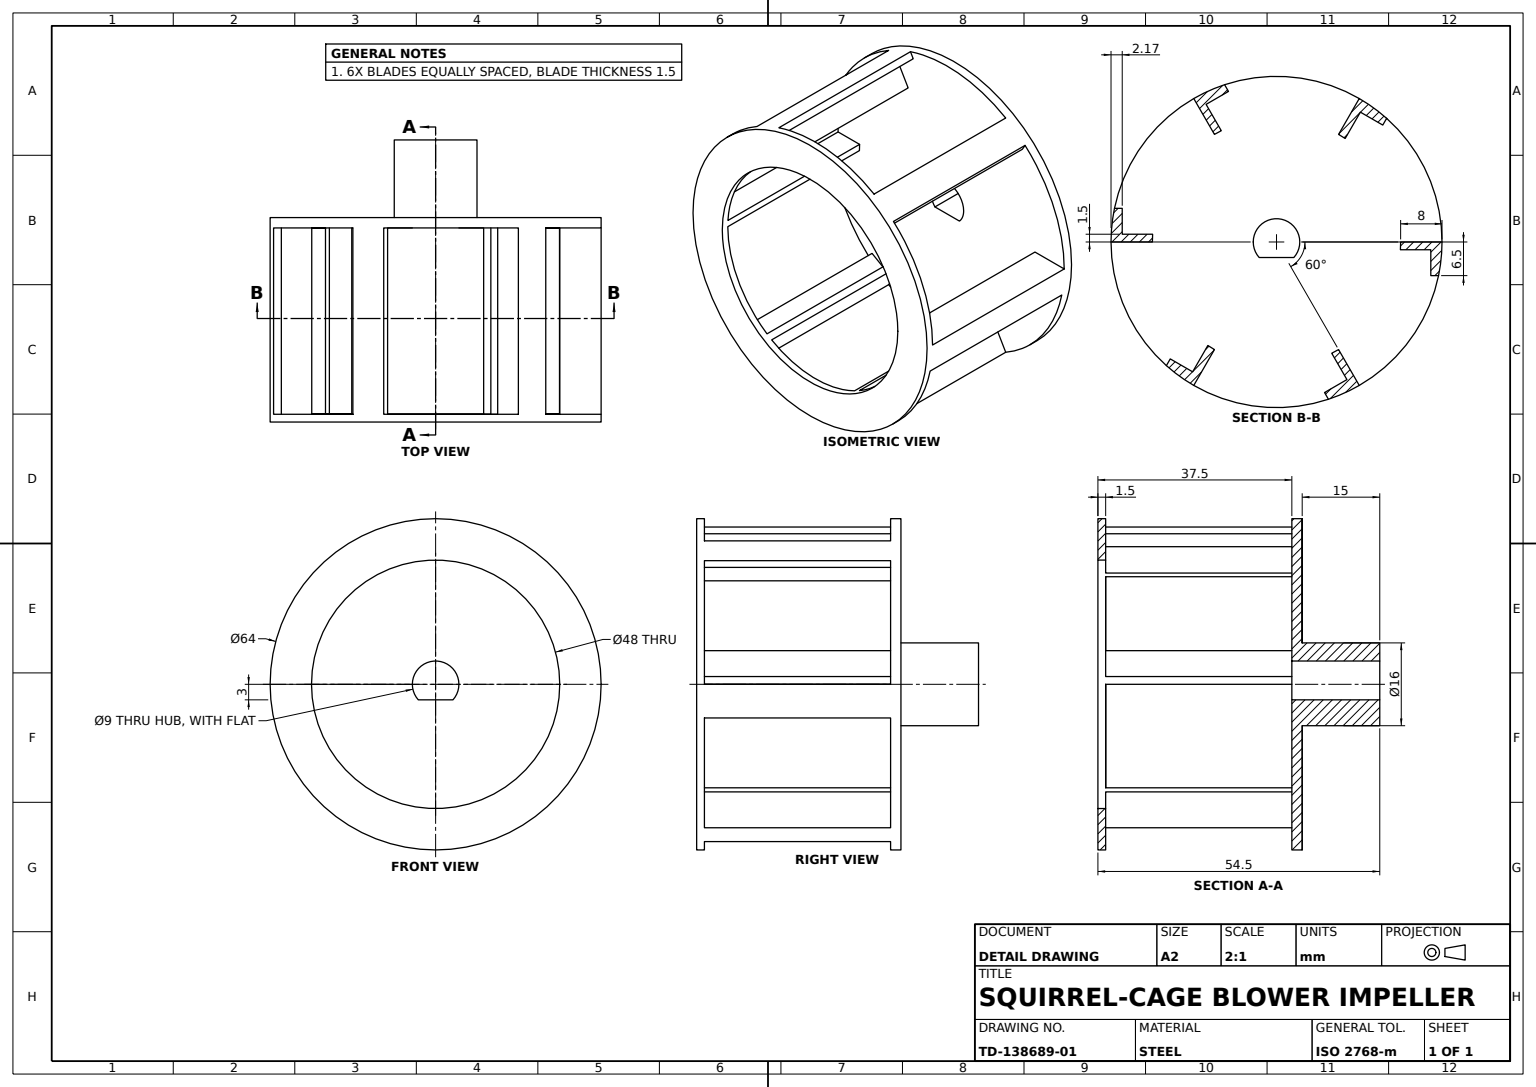
ISO-10303-21;
HEADER;
FILE_DESCRIPTION((''),'2;1');
FILE_NAME('','',(''),(''),'','','');
FILE_SCHEMA(('AUTOMOTIVE_DESIGN'));
ENDSEC;
DATA;
#1=APPLICATION_CONTEXT('');
#2=PRODUCT_CONTEXT('',#1,'mechanical');
#3=PRODUCT('','','',(#2));
#4=PRODUCT_DEFINITION_FORMATION('','',#3);
#5=PRODUCT_DEFINITION_CONTEXT('',#1,'design');
#6=PRODUCT_DEFINITION('','',#4,#5);
#7=PRODUCT_DEFINITION_SHAPE('','',#6);
#8=(LENGTH_UNIT()NAMED_UNIT(*)SI_UNIT(.MILLI.,.METRE.));
#9=(NAMED_UNIT(*)PLANE_ANGLE_UNIT()SI_UNIT($,.RADIAN.));
#10=(NAMED_UNIT(*)SI_UNIT($,.STERADIAN.)SOLID_ANGLE_UNIT());
#11=UNCERTAINTY_MEASURE_WITH_UNIT(LENGTH_MEASURE(1.E-05),#8,'distance_accuracy_value','');
#12=(GEOMETRIC_REPRESENTATION_CONTEXT(3)GLOBAL_UNCERTAINTY_ASSIGNED_CONTEXT((#11))GLOBAL_UNIT_ASSIGNED_CONTEXT((#8,#9,#10))REPRESENTATION_CONTEXT('',''));
#13=CARTESIAN_POINT('',(13.617407,-26.586041,38.));
#14=VERTEX_POINT('',#13);
#15=CARTESIAN_POINT('',(13.617407,-26.586041,2.));
#16=VERTEX_POINT('',#15);
#17=CARTESIAN_POINT('',(13.617407,-26.586041,39.5));
#18=DIRECTION('',(0.,0.,-1.));
#19=VECTOR('',#18,1000.);
#20=LINE('',#17,#19);
#21=EDGE_CURVE('',#14,#16,#20,.T.);
#22=ORIENTED_EDGE('',*,*,#21,.T.);
#23=CARTESIAN_POINT('',(9.28728,-29.086041,2.));
#24=VERTEX_POINT('',#23);
#25=DIRECTION('',(-0.866025404,-0.5,0.));
#26=VECTOR('',#25,1000.);
#27=LINE('',#15,#26);
#28=EDGE_CURVE('',#16,#24,#27,.T.);
#29=ORIENTED_EDGE('',*,*,#28,.T.);
#30=CARTESIAN_POINT('',(9.28728,-29.086041,38.));
#31=VERTEX_POINT('',#30);
#32=CARTESIAN_POINT('',(9.28728,-29.086041,39.5));
#33=LINE('',#32,#19);
#34=EDGE_CURVE('',#31,#24,#33,.T.);
#35=ORIENTED_EDGE('',*,*,#34,.F.);
#36=LINE('',#13,#26);
#37=EDGE_CURVE('',#14,#31,#36,.T.);
#38=ORIENTED_EDGE('',*,*,#37,.F.);
#39=EDGE_LOOP('',(#22,#29,#35,#38));
#40=FACE_OUTER_BOUND('',#39,.T.);
#41=DIRECTION('',(0.5,-0.866025404,0.));
#42=DIRECTION('',(0.866025404,0.5,0.));
#43=AXIS2_PLACEMENT_3D('',#17,#41,#42);
#44=PLANE('',#43);
#45=ADVANCED_FACE('',(#40),#44,.F.);
#46=CARTESIAN_POINT('',(20.54561,22.586041,38.));
#47=VERTEX_POINT('',#46);
#48=CARTESIAN_POINT('',(20.54561,22.586041,2.));
#49=VERTEX_POINT('',#48);
#50=CARTESIAN_POINT('',(20.54561,22.586041,39.5));
#51=LINE('',#50,#19);
#52=EDGE_CURVE('',#47,#49,#51,.T.);
#53=ORIENTED_EDGE('',*,*,#52,.T.);
#54=CARTESIAN_POINT('',(21.29561,23.885079,2.));
#55=VERTEX_POINT('',#54);
#56=DIRECTION('',(0.5,0.866025404,0.));
#57=VECTOR('',#56,1000.);
#58=LINE('',#48,#57);
#59=EDGE_CURVE('',#49,#55,#58,.T.);
#60=ORIENTED_EDGE('',*,*,#59,.T.);
#61=CARTESIAN_POINT('',(21.29561,23.885079,38.));
#62=VERTEX_POINT('',#61);
#63=CARTESIAN_POINT('',(21.29561,23.885079,39.5));
#64=LINE('',#63,#19);
#65=EDGE_CURVE('',#62,#55,#64,.T.);
#66=ORIENTED_EDGE('',*,*,#65,.F.);
#67=LINE('',#46,#57);
#68=EDGE_CURVE('',#47,#62,#67,.T.);
#69=ORIENTED_EDGE('',*,*,#68,.F.);
#70=EDGE_LOOP('',(#53,#60,#66,#69));
#71=FACE_OUTER_BOUND('',#70,.T.);
#72=DIRECTION('',(-0.866025404,0.5,0.));
#73=DIRECTION('',(-0.5,-0.866025404,0.));
#74=AXIS2_PLACEMENT_3D('',#50,#72,#73);
#75=PLANE('',#74);
#76=ADVANCED_FACE('',(#71),#75,.F.);
#77=CARTESIAN_POINT('',(-12.,20.78461,38.));
#78=VERTEX_POINT('',#77);
#79=CARTESIAN_POINT('',(-23.953079,1.5,38.));
#80=VERTEX_POINT('',#79);
#81=CARTESIAN_POINT('',(0.,0.,38.));
#82=DIRECTION('',(0.,0.,1.));
#83=DIRECTION('',(1.,0.,0.));
#84=AXIS2_PLACEMENT_3D('',#81,#82,#83);
#85=CIRCLE('',#84,24.);
#86=EDGE_CURVE('',#78,#80,#85,.T.);
#87=ORIENTED_EDGE('',*,*,#86,.T.);
#88=CARTESIAN_POINT('',(-29.83289,1.5,38.));
#89=VERTEX_POINT('',#88);
#90=DIRECTION('',(-1.,0.,0.));
#91=VECTOR('',#90,1000.);
#92=LINE('',#79,#91);
#93=EDGE_CURVE('',#80,#89,#92,.T.);
#94=ORIENTED_EDGE('',*,*,#93,.T.);
#95=CARTESIAN_POINT('',(-29.83289,6.5,38.));
#96=VERTEX_POINT('',#95);
#97=DIRECTION('',(0.,1.,0.));
#98=VECTOR('',#97,1000.);
#99=LINE('',#88,#98);
#100=EDGE_CURVE('',#89,#96,#99,.T.);
#101=ORIENTED_EDGE('',*,*,#100,.T.);
#102=CARTESIAN_POINT('',(-31.33289,6.5,38.));
#103=VERTEX_POINT('',#102);
#104=LINE('',#95,#91);
#105=EDGE_CURVE('',#96,#103,#104,.T.);
#106=ORIENTED_EDGE('',*,*,#105,.T.);
#107=CARTESIAN_POINT('',(-16.,27.712813,38.));
#108=VERTEX_POINT('',#107);
#109=CIRCLE('',#84,32.);
#110=EDGE_CURVE('',#108,#103,#109,.T.);
#111=ORIENTED_EDGE('',*,*,#110,.F.);
#112=VECTOR('',#41,1000.);
#113=LINE('',#107,#112);
#114=EDGE_CURVE('',#108,#78,#113,.T.);
#115=ORIENTED_EDGE('',*,*,#114,.T.);
#116=EDGE_LOOP('',(#87,#94,#101,#106,#111,#115));
#117=FACE_OUTER_BOUND('',#116,.T.);
#118=PLANE('',#84);
#119=ADVANCED_FACE('',(#117),#118,.F.);
#120=CARTESIAN_POINT('',(10.677501,-21.493975,2.));
#121=VERTEX_POINT('',#120);
#122=LINE('',#120,#112);
#123=EDGE_CURVE('',#121,#16,#122,.T.);
#124=ORIENTED_EDGE('',*,*,#123,.T.);
#125=ORIENTED_EDGE('',*,*,#21,.F.);
#126=CARTESIAN_POINT('',(10.677501,-21.493975,38.));
#127=VERTEX_POINT('',#126);
#128=LINE('',#126,#112);
#129=EDGE_CURVE('',#127,#14,#128,.T.);
#130=ORIENTED_EDGE('',*,*,#129,.F.);
#131=CARTESIAN_POINT('',(10.677501,-21.493975,39.5));
#132=LINE('',#131,#19);
#133=EDGE_CURVE('',#127,#121,#132,.T.);
#134=ORIENTED_EDGE('',*,*,#133,.T.);
#135=EDGE_LOOP('',(#124,#125,#130,#134));
#136=FACE_OUTER_BOUND('',#135,.T.);
#137=DIRECTION('',(-0.5,0.866025404,0.));
#138=AXIS2_PLACEMENT_3D('',#131,#42,#137);
#139=PLANE('',#138);
#140=ADVANCED_FACE('',(#136),#139,.F.);
#141=CARTESIAN_POINT('',(16.,27.712813,38.));
#142=VERTEX_POINT('',#141);
#143=CARTESIAN_POINT('',(16.,27.712813,2.));
#144=VERTEX_POINT('',#143);
#145=CARTESIAN_POINT('',(16.,27.712813,39.5));
#146=LINE('',#145,#19);
#147=EDGE_CURVE('',#142,#144,#146,.T.);
#148=ORIENTED_EDGE('',*,*,#147,.T.);
#149=CARTESIAN_POINT('',(12.,20.78461,2.));
#150=VERTEX_POINT('',#149);
#151=VECTOR('',#73,1000.);
#152=LINE('',#143,#151);
#153=EDGE_CURVE('',#144,#150,#152,.T.);
#154=ORIENTED_EDGE('',*,*,#153,.T.);
#155=CARTESIAN_POINT('',(12.,20.78461,38.));
#156=VERTEX_POINT('',#155);
#157=CARTESIAN_POINT('',(12.,20.78461,39.5));
#158=LINE('',#157,#19);
#159=EDGE_CURVE('',#156,#150,#158,.T.);
#160=ORIENTED_EDGE('',*,*,#159,.F.);
#161=LINE('',#141,#151);
#162=EDGE_CURVE('',#142,#156,#161,.T.);
#163=ORIENTED_EDGE('',*,*,#162,.F.);
#164=EDGE_LOOP('',(#148,#154,#160,#163));
#165=FACE_OUTER_BOUND('',#164,.T.);
#166=DIRECTION('',(0.866025404,-0.5,0.));
#167=AXIS2_PLACEMENT_3D('',#145,#166,#56);
#168=PLANE('',#167);
#169=ADVANCED_FACE('',(#165),#168,.F.);
#170=CARTESIAN_POINT('',(-10.03728,30.385079,38.));
#171=VERTEX_POINT('',#170);
#172=EDGE_CURVE('',#142,#171,#109,.T.);
#173=ORIENTED_EDGE('',*,*,#172,.F.);
#174=ORIENTED_EDGE('',*,*,#162,.T.);
#175=CARTESIAN_POINT('',(-10.677501,21.493975,38.));
#176=VERTEX_POINT('',#175);
#177=EDGE_CURVE('',#156,#176,#85,.T.);
#178=ORIENTED_EDGE('',*,*,#177,.T.);
#179=CARTESIAN_POINT('',(-13.617407,26.586041,38.));
#180=VERTEX_POINT('',#179);
#181=VECTOR('',#137,1000.);
#182=LINE('',#175,#181);
#183=EDGE_CURVE('',#176,#180,#182,.T.);
#184=ORIENTED_EDGE('',*,*,#183,.T.);
#185=CARTESIAN_POINT('',(-9.28728,29.086041,38.));
#186=VERTEX_POINT('',#185);
#187=VECTOR('',#42,1000.);
#188=LINE('',#179,#187);
#189=EDGE_CURVE('',#180,#186,#188,.T.);
#190=ORIENTED_EDGE('',*,*,#189,.T.);
#191=LINE('',#185,#181);
#192=EDGE_CURVE('',#186,#171,#191,.T.);
#193=ORIENTED_EDGE('',*,*,#192,.T.);
#194=EDGE_LOOP('',(#173,#174,#178,#184,#190,#193));
#195=FACE_OUTER_BOUND('',#194,.T.);
#196=ADVANCED_FACE('',(#195),#118,.F.);
#197=CARTESIAN_POINT('',(-32.,0.,2.));
#198=VERTEX_POINT('',#197);
#199=CARTESIAN_POINT('',(-24.,0.,2.));
#200=VERTEX_POINT('',#199);
#201=VECTOR('',#83,1000.);
#202=LINE('',#197,#201);
#203=EDGE_CURVE('',#198,#200,#202,.T.);
#204=ORIENTED_EDGE('',*,*,#203,.T.);
#205=CARTESIAN_POINT('',(-24.,0.,38.));
#206=VERTEX_POINT('',#205);
#207=CARTESIAN_POINT('',(-24.,0.,39.5));
#208=LINE('',#207,#19);
#209=EDGE_CURVE('',#206,#200,#208,.T.);
#210=ORIENTED_EDGE('',*,*,#209,.F.);
#211=CARTESIAN_POINT('',(-32.,0.,38.));
#212=VERTEX_POINT('',#211);
#213=LINE('',#211,#201);
#214=EDGE_CURVE('',#212,#206,#213,.T.);
#215=ORIENTED_EDGE('',*,*,#214,.F.);
#216=CARTESIAN_POINT('',(-32.,0.,39.5));
#217=LINE('',#216,#19);
#218=EDGE_CURVE('',#212,#198,#217,.T.);
#219=ORIENTED_EDGE('',*,*,#218,.T.);
#220=EDGE_LOOP('',(#204,#210,#215,#219));
#221=FACE_OUTER_BOUND('',#220,.T.);
#222=AXIS2_PLACEMENT_3D('',#216,#97,#90);
#223=PLANE('',#222);
#224=ADVANCED_FACE('',(#221),#223,.F.);
#225=CARTESIAN_POINT('',(-23.953079,1.5,2.));
#226=VERTEX_POINT('',#225);
#227=CARTESIAN_POINT('',(-23.953079,1.5,39.5));
#228=LINE('',#227,#19);
#229=EDGE_CURVE('',#80,#226,#228,.T.);
#230=ORIENTED_EDGE('',*,*,#229,.T.);
#231=CARTESIAN_POINT('',(-29.83289,1.5,2.));
#232=VERTEX_POINT('',#231);
#233=LINE('',#225,#91);
#234=EDGE_CURVE('',#226,#232,#233,.T.);
#235=ORIENTED_EDGE('',*,*,#234,.T.);
#236=CARTESIAN_POINT('',(-29.83289,1.5,39.5));
#237=LINE('',#236,#19);
#238=EDGE_CURVE('',#89,#232,#237,.T.);
#239=ORIENTED_EDGE('',*,*,#238,.F.);
#240=ORIENTED_EDGE('',*,*,#93,.F.);
#241=EDGE_LOOP('',(#230,#235,#239,#240));
#242=FACE_OUTER_BOUND('',#241,.T.);
#243=DIRECTION('',(0.,-1.,0.));
#244=AXIS2_PLACEMENT_3D('',#227,#243,#83);
#245=PLANE('',#244);
#246=ADVANCED_FACE('',(#242),#245,.F.);
#247=CARTESIAN_POINT('',(16.215483,25.086041,38.));
#248=VERTEX_POINT('',#247);
#249=CARTESIAN_POINT('',(16.215483,25.086041,2.));
#250=VERTEX_POINT('',#249);
#251=CARTESIAN_POINT('',(16.215483,25.086041,39.5));
#252=LINE('',#251,#19);
#253=EDGE_CURVE('',#248,#250,#252,.T.);
#254=ORIENTED_EDGE('',*,*,#253,.T.);
#255=VECTOR('',#166,1000.);
#256=LINE('',#249,#255);
#257=EDGE_CURVE('',#250,#49,#256,.T.);
#258=ORIENTED_EDGE('',*,*,#257,.T.);
#259=ORIENTED_EDGE('',*,*,#52,.F.);
#260=LINE('',#247,#255);
#261=EDGE_CURVE('',#248,#47,#260,.T.);
#262=ORIENTED_EDGE('',*,*,#261,.F.);
#263=EDGE_LOOP('',(#254,#258,#259,#262));
#264=FACE_OUTER_BOUND('',#263,.T.);
#265=AXIS2_PLACEMENT_3D('',#251,#56,#72);
#266=PLANE('',#265);
#267=ADVANCED_FACE('',(#264),#266,.F.);
#268=CARTESIAN_POINT('',(3.354102,-3.,-15.));
#269=VERTEX_POINT('',#268);
#270=CARTESIAN_POINT('',(3.354102,-3.,2.));
#271=VERTEX_POINT('',#270);
#272=VECTOR('',#82,1000.);
#273=LINE('',#268,#272);
#274=EDGE_CURVE('',#269,#271,#273,.T.);
#275=ORIENTED_EDGE('',*,*,#274,.T.);
#276=CARTESIAN_POINT('',(4.5,0.,2.));
#277=VERTEX_POINT('',#276);
#278=CARTESIAN_POINT('',(0.,0.,2.));
#279=AXIS2_PLACEMENT_3D('',#278,#82,#83);
#280=CIRCLE('',#279,4.5);
#281=EDGE_CURVE('',#271,#277,#280,.T.);
#282=ORIENTED_EDGE('',*,*,#281,.T.);
#283=CARTESIAN_POINT('',(4.5,0.,-15.));
#284=VERTEX_POINT('',#283);
#285=LINE('',#283,#272);
#286=EDGE_CURVE('',#284,#277,#285,.T.);
#287=ORIENTED_EDGE('',*,*,#286,.F.);
#288=CARTESIAN_POINT('',(0.,0.,-15.));
#289=AXIS2_PLACEMENT_3D('',#288,#18,#90);
#290=CIRCLE('',#289,4.5);
#291=EDGE_CURVE('',#284,#269,#290,.T.);
#292=ORIENTED_EDGE('',*,*,#291,.T.);
#293=EDGE_LOOP('',(#275,#282,#287,#292));
#294=FACE_OUTER_BOUND('',#293,.T.);
#295=AXIS2_PLACEMENT_3D('',#288,#82,#83);
#296=CYLINDRICAL_SURFACE('',#295,4.5);
#297=ADVANCED_FACE('',(#294),#296,.F.);
#298=CARTESIAN_POINT('',(-9.28728,29.086041,2.));
#299=VERTEX_POINT('',#298);
#300=CARTESIAN_POINT('',(-9.28728,29.086041,39.5));
#301=LINE('',#300,#19);
#302=EDGE_CURVE('',#186,#299,#301,.T.);
#303=ORIENTED_EDGE('',*,*,#302,.T.);
#304=CARTESIAN_POINT('',(-10.03728,30.385079,2.));
#305=VERTEX_POINT('',#304);
#306=LINE('',#298,#181);
#307=EDGE_CURVE('',#299,#305,#306,.T.);
#308=ORIENTED_EDGE('',*,*,#307,.T.);
#309=CARTESIAN_POINT('',(-10.03728,30.385079,39.5));
#310=LINE('',#309,#19);
#311=EDGE_CURVE('',#171,#305,#310,.T.);
#312=ORIENTED_EDGE('',*,*,#311,.F.);
#313=ORIENTED_EDGE('',*,*,#192,.F.);
#314=EDGE_LOOP('',(#303,#308,#312,#313));
#315=FACE_OUTER_BOUND('',#314,.T.);
#316=AXIS2_PLACEMENT_3D('',#300,#25,#41);
#317=PLANE('',#316);
#318=ADVANCED_FACE('',(#315),#317,.F.);
#319=CARTESIAN_POINT('',(-21.29561,-23.885079,38.));
#320=VERTEX_POINT('',#319);
#321=EDGE_CURVE('',#212,#320,#109,.T.);
#322=ORIENTED_EDGE('',*,*,#321,.T.);
#323=CARTESIAN_POINT('',(-21.29561,-23.885079,2.));
#324=VERTEX_POINT('',#323);
#325=CARTESIAN_POINT('',(-21.29561,-23.885079,39.5));
#326=LINE('',#325,#19);
#327=EDGE_CURVE('',#320,#324,#326,.T.);
#328=ORIENTED_EDGE('',*,*,#327,.T.);
#329=CIRCLE('',#279,32.);
#330=EDGE_CURVE('',#198,#324,#329,.T.);
#331=ORIENTED_EDGE('',*,*,#330,.F.);
#332=CARTESIAN_POINT('',(-32.,0.,0.));
#333=VERTEX_POINT('',#332);
#334=LINE('',#197,#19);
#335=EDGE_CURVE('',#198,#333,#334,.T.);
#336=ORIENTED_EDGE('',*,*,#335,.T.);
#337=CARTESIAN_POINT('',(32.,0.,0.));
#338=VERTEX_POINT('',#337);
#339=CARTESIAN_POINT('',(0.,0.,0.));
#340=AXIS2_PLACEMENT_3D('',#339,#82,#83);
#341=CIRCLE('',#340,32.);
#342=EDGE_CURVE('',#333,#338,#341,.T.);
#343=ORIENTED_EDGE('',*,*,#342,.T.);
#344=CARTESIAN_POINT('',(32.,0.,2.));
#345=VERTEX_POINT('',#344);
#346=LINE('',#344,#19);
#347=EDGE_CURVE('',#345,#338,#346,.T.);
#348=ORIENTED_EDGE('',*,*,#347,.F.);
#349=CARTESIAN_POINT('',(32.,0.,38.));
#350=VERTEX_POINT('',#349);
#351=CARTESIAN_POINT('',(32.,0.,39.5));
#352=LINE('',#351,#19);
#353=EDGE_CURVE('',#350,#345,#352,.T.);
#354=ORIENTED_EDGE('',*,*,#353,.F.);
#355=VERTEX_POINT('',#351);
#356=EDGE_CURVE('',#355,#350,#346,.T.);
#357=ORIENTED_EDGE('',*,*,#356,.F.);
#358=VERTEX_POINT('',#216);
#359=CARTESIAN_POINT('',(0.,0.,39.5));
#360=AXIS2_PLACEMENT_3D('',#359,#82,#83);
#361=CIRCLE('',#360,32.);
#362=EDGE_CURVE('',#358,#355,#361,.T.);
#363=ORIENTED_EDGE('',*,*,#362,.F.);
#364=EDGE_CURVE('',#358,#212,#334,.T.);
#365=ORIENTED_EDGE('',*,*,#364,.T.);
#366=EDGE_LOOP('',(#322,#328,#331,#336,#343,#348,#354,#357,#363,#365));
#367=FACE_OUTER_BOUND('',#366,.T.);
#368=CARTESIAN_POINT('',(-16.,-27.712813,2.));
#369=VERTEX_POINT('',#368);
#370=CARTESIAN_POINT('',(10.03728,-30.385079,2.));
#371=VERTEX_POINT('',#370);
#372=EDGE_CURVE('',#369,#371,#329,.T.);
#373=ORIENTED_EDGE('',*,*,#372,.F.);
#374=CARTESIAN_POINT('',(-16.,-27.712813,38.));
#375=VERTEX_POINT('',#374);
#376=CARTESIAN_POINT('',(-16.,-27.712813,39.5));
#377=LINE('',#376,#19);
#378=EDGE_CURVE('',#375,#369,#377,.T.);
#379=ORIENTED_EDGE('',*,*,#378,.F.);
#380=CARTESIAN_POINT('',(10.03728,-30.385079,38.));
#381=VERTEX_POINT('',#380);
#382=EDGE_CURVE('',#375,#381,#109,.T.);
#383=ORIENTED_EDGE('',*,*,#382,.T.);
#384=CARTESIAN_POINT('',(10.03728,-30.385079,39.5));
#385=LINE('',#384,#19);
#386=EDGE_CURVE('',#381,#371,#385,.T.);
#387=ORIENTED_EDGE('',*,*,#386,.T.);
#388=EDGE_LOOP('',(#373,#379,#383,#387));
#389=FACE_BOUND('',#388,.T.);
#390=CARTESIAN_POINT('',(16.,-27.712813,38.));
#391=VERTEX_POINT('',#390);
#392=CARTESIAN_POINT('',(31.33289,-6.5,38.));
#393=VERTEX_POINT('',#392);
#394=EDGE_CURVE('',#391,#393,#109,.T.);
#395=ORIENTED_EDGE('',*,*,#394,.T.);
#396=CARTESIAN_POINT('',(31.33289,-6.5,2.));
#397=VERTEX_POINT('',#396);
#398=CARTESIAN_POINT('',(31.33289,-6.5,39.5));
#399=LINE('',#398,#19);
#400=EDGE_CURVE('',#393,#397,#399,.T.);
#401=ORIENTED_EDGE('',*,*,#400,.T.);
#402=CARTESIAN_POINT('',(16.,-27.712813,2.));
#403=VERTEX_POINT('',#402);
#404=EDGE_CURVE('',#403,#397,#329,.T.);
#405=ORIENTED_EDGE('',*,*,#404,.F.);
#406=CARTESIAN_POINT('',(16.,-27.712813,39.5));
#407=LINE('',#406,#19);
#408=EDGE_CURVE('',#391,#403,#407,.T.);
#409=ORIENTED_EDGE('',*,*,#408,.F.);
#410=EDGE_LOOP('',(#395,#401,#405,#409));
#411=FACE_BOUND('',#410,.T.);
#412=AXIS2_PLACEMENT_3D('',#278,#18,#90);
#413=CYLINDRICAL_SURFACE('',#412,32.);
#414=ADVANCED_FACE('',(#367,#389,#411),#413,.T.);
#415=CARTESIAN_POINT('',(-10.677501,21.493975,2.));
#416=VERTEX_POINT('',#415);
#417=CARTESIAN_POINT('',(-10.677501,21.493975,39.5));
#418=LINE('',#417,#19);
#419=EDGE_CURVE('',#176,#416,#418,.T.);
#420=ORIENTED_EDGE('',*,*,#419,.T.);
#421=CARTESIAN_POINT('',(-13.617407,26.586041,2.));
#422=VERTEX_POINT('',#421);
#423=LINE('',#415,#181);
#424=EDGE_CURVE('',#416,#422,#423,.T.);
#425=ORIENTED_EDGE('',*,*,#424,.T.);
#426=CARTESIAN_POINT('',(-13.617407,26.586041,39.5));
#427=LINE('',#426,#19);
#428=EDGE_CURVE('',#180,#422,#427,.T.);
#429=ORIENTED_EDGE('',*,*,#428,.F.);
#430=ORIENTED_EDGE('',*,*,#183,.F.);
#431=EDGE_LOOP('',(#420,#425,#429,#430));
#432=FACE_OUTER_BOUND('',#431,.T.);
#433=AXIS2_PLACEMENT_3D('',#417,#25,#41);
#434=PLANE('',#433);
#435=ADVANCED_FACE('',(#432),#434,.F.);
#436=CARTESIAN_POINT('',(-3.354102,-3.,-15.));
#437=VERTEX_POINT('',#436);
#438=LINE('',#436,#201);
#439=EDGE_CURVE('',#437,#269,#438,.T.);
#440=ORIENTED_EDGE('',*,*,#439,.F.);
#441=CARTESIAN_POINT('',(-3.354102,-3.,0.));
#442=VERTEX_POINT('',#441);
#443=LINE('',#436,#272);
#444=EDGE_CURVE('',#437,#442,#443,.T.);
#445=ORIENTED_EDGE('',*,*,#444,.T.);
#446=CARTESIAN_POINT('',(-3.354102,-3.,2.));
#447=VERTEX_POINT('',#446);
#448=CARTESIAN_POINT('',(-3.354102,-3.,15.));
#449=LINE('',#448,#19);
#450=EDGE_CURVE('',#447,#442,#449,.T.);
#451=ORIENTED_EDGE('',*,*,#450,.F.);
#452=CARTESIAN_POINT('',(0.,-3.,2.));
#453=LINE('',#452,#201);
#454=EDGE_CURVE('',#447,#271,#453,.T.);
#455=ORIENTED_EDGE('',*,*,#454,.T.);
#456=ORIENTED_EDGE('',*,*,#274,.F.);
#457=EDGE_LOOP('',(#440,#445,#451,#455,#456));
#458=FACE_OUTER_BOUND('',#457,.T.);
#459=AXIS2_PLACEMENT_3D('',#436,#243,#18);
#460=PLANE('',#459);
#461=ADVANCED_FACE('',(#458),#460,.F.);
#462=ORIENTED_EDGE('',*,*,#353,.T.);
#463=CARTESIAN_POINT('',(24.,0.,2.));
#464=VERTEX_POINT('',#463);
#465=LINE('',#344,#91);
#466=EDGE_CURVE('',#345,#464,#465,.T.);
#467=ORIENTED_EDGE('',*,*,#466,.T.);
#468=CARTESIAN_POINT('',(24.,0.,38.));
#469=VERTEX_POINT('',#468);
#470=CARTESIAN_POINT('',(24.,0.,39.5));
#471=LINE('',#470,#19);
#472=EDGE_CURVE('',#469,#464,#471,.T.);
#473=ORIENTED_EDGE('',*,*,#472,.F.);
#474=LINE('',#349,#91);
#475=EDGE_CURVE('',#350,#469,#474,.T.);
#476=ORIENTED_EDGE('',*,*,#475,.F.);
#477=EDGE_LOOP('',(#462,#467,#473,#476));
#478=FACE_OUTER_BOUND('',#477,.T.);
#479=AXIS2_PLACEMENT_3D('',#351,#243,#83);
#480=PLANE('',#479);
#481=ADVANCED_FACE('',(#478),#480,.F.);
#482=ORIENTED_EDGE('',*,*,#105,.F.);
#483=CARTESIAN_POINT('',(-29.83289,6.5,2.));
#484=VERTEX_POINT('',#483);
#485=CARTESIAN_POINT('',(-29.83289,6.5,39.5));
#486=LINE('',#485,#19);
#487=EDGE_CURVE('',#96,#484,#486,.T.);
#488=ORIENTED_EDGE('',*,*,#487,.T.);
#489=CARTESIAN_POINT('',(-31.33289,6.5,2.));
#490=VERTEX_POINT('',#489);
#491=LINE('',#483,#91);
#492=EDGE_CURVE('',#484,#490,#491,.T.);
#493=ORIENTED_EDGE('',*,*,#492,.T.);
#494=CARTESIAN_POINT('',(-31.33289,6.5,39.5));
#495=LINE('',#494,#19);
#496=EDGE_CURVE('',#103,#490,#495,.T.);
#497=ORIENTED_EDGE('',*,*,#496,.F.);
#498=EDGE_LOOP('',(#482,#488,#493,#497));
#499=FACE_OUTER_BOUND('',#498,.T.);
#500=AXIS2_PLACEMENT_3D('',#485,#243,#83);
#501=PLANE('',#500);
#502=ADVANCED_FACE('',(#499),#501,.F.);
#503=CARTESIAN_POINT('',(23.953079,-1.5,38.));
#504=VERTEX_POINT('',#503);
#505=CARTESIAN_POINT('',(23.953079,-1.5,2.));
#506=VERTEX_POINT('',#505);
#507=CARTESIAN_POINT('',(23.953079,-1.5,39.5));
#508=LINE('',#507,#19);
#509=EDGE_CURVE('',#504,#506,#508,.T.);
#510=ORIENTED_EDGE('',*,*,#509,.F.);
#511=CARTESIAN_POINT('',(12.,-20.78461,38.));
#512=VERTEX_POINT('',#511);
#513=EDGE_CURVE('',#512,#504,#85,.T.);
#514=ORIENTED_EDGE('',*,*,#513,.F.);
#515=CARTESIAN_POINT('',(12.,-20.78461,2.));
#516=VERTEX_POINT('',#515);
#517=CARTESIAN_POINT('',(12.,-20.78461,39.5));
#518=LINE('',#517,#19);
#519=EDGE_CURVE('',#512,#516,#518,.T.);
#520=ORIENTED_EDGE('',*,*,#519,.T.);
#521=AXIS2_PLACEMENT_3D('',#278,#18,#83);
#522=CIRCLE('',#521,24.);
#523=EDGE_CURVE('',#516,#121,#522,.T.);
#524=ORIENTED_EDGE('',*,*,#523,.T.);
#525=ORIENTED_EDGE('',*,*,#133,.F.);
#526=CARTESIAN_POINT('',(-12.,-20.78461,38.));
#527=VERTEX_POINT('',#526);
#528=EDGE_CURVE('',#527,#127,#85,.T.);
#529=ORIENTED_EDGE('',*,*,#528,.F.);
#530=CARTESIAN_POINT('',(-12.,-20.78461,2.));
#531=VERTEX_POINT('',#530);
#532=CARTESIAN_POINT('',(-12.,-20.78461,39.5));
#533=LINE('',#532,#19);
#534=EDGE_CURVE('',#527,#531,#533,.T.);
#535=ORIENTED_EDGE('',*,*,#534,.T.);
#536=CARTESIAN_POINT('',(-13.275578,-19.993975,2.));
#537=VERTEX_POINT('',#536);
#538=EDGE_CURVE('',#531,#537,#522,.T.);
#539=ORIENTED_EDGE('',*,*,#538,.T.);
#540=CARTESIAN_POINT('',(-13.275578,-19.993975,38.));
#541=VERTEX_POINT('',#540);
#542=CARTESIAN_POINT('',(-13.275578,-19.993975,39.5));
#543=LINE('',#542,#19);
#544=EDGE_CURVE('',#541,#537,#543,.T.);
#545=ORIENTED_EDGE('',*,*,#544,.F.);
#546=EDGE_CURVE('',#206,#541,#85,.T.);
#547=ORIENTED_EDGE('',*,*,#546,.F.);
#548=VERTEX_POINT('',#207);
#549=EDGE_CURVE('',#548,#206,#208,.T.);
#550=ORIENTED_EDGE('',*,*,#549,.F.);
#551=VERTEX_POINT('',#470);
#552=AXIS2_PLACEMENT_3D('',#359,#18,#83);
#553=CIRCLE('',#552,24.);
#554=EDGE_CURVE('',#551,#548,#553,.T.);
#555=ORIENTED_EDGE('',*,*,#554,.F.);
#556=EDGE_CURVE('',#551,#469,#471,.T.);
#557=ORIENTED_EDGE('',*,*,#556,.T.);
#558=ORIENTED_EDGE('',*,*,#472,.T.);
#559=EDGE_CURVE('',#464,#506,#522,.T.);
#560=ORIENTED_EDGE('',*,*,#559,.T.);
#561=EDGE_LOOP('',(#510,#514,#520,#524,#525,#529,#535,#539,#545,#547,#550,#555,#557,#558,#560));
#562=FACE_OUTER_BOUND('',#561,.T.);
#563=AXIS2_PLACEMENT_3D('',#359,#18,#90);
#564=CYLINDRICAL_SURFACE('',#563,24.);
#565=ADVANCED_FACE('',(#562),#564,.F.);
#566=EDGE_CURVE('',#338,#333,#341,.T.);
#567=ORIENTED_EDGE('',*,*,#566,.F.);
#568=ORIENTED_EDGE('',*,*,#342,.F.);
#569=EDGE_LOOP('',(#567,#568));
#570=FACE_OUTER_BOUND('',#569,.T.);
#571=CARTESIAN_POINT('',(-8.,0.,0.));
#572=VERTEX_POINT('',#571);
#573=CARTESIAN_POINT('',(8.,0.,0.));
#574=VERTEX_POINT('',#573);
#575=AXIS2_PLACEMENT_3D('',#339,#18,#90);
#576=CIRCLE('',#575,8.);
#577=EDGE_CURVE('',#572,#574,#576,.T.);
#578=ORIENTED_EDGE('',*,*,#577,.F.);
#579=EDGE_CURVE('',#574,#572,#576,.T.);
#580=ORIENTED_EDGE('',*,*,#579,.F.);
#581=EDGE_LOOP('',(#578,#580));
#582=FACE_BOUND('',#581,.T.);
#583=PLANE('',#340);
#584=ADVANCED_FACE('',(#570,#582),#583,.F.);
#585=CARTESIAN_POINT('',(-4.5,0.,-15.));
#586=VERTEX_POINT('',#585);
#587=EDGE_CURVE('',#586,#284,#290,.T.);
#588=ORIENTED_EDGE('',*,*,#587,.T.);
#589=ORIENTED_EDGE('',*,*,#286,.T.);
#590=CARTESIAN_POINT('',(-4.5,0.,2.));
#591=VERTEX_POINT('',#590);
#592=EDGE_CURVE('',#277,#591,#280,.T.);
#593=ORIENTED_EDGE('',*,*,#592,.T.);
#594=LINE('',#585,#272);
#595=EDGE_CURVE('',#586,#591,#594,.T.);
#596=ORIENTED_EDGE('',*,*,#595,.F.);
#597=EDGE_LOOP('',(#588,#589,#593,#596));
#598=FACE_OUTER_BOUND('',#597,.T.);
#599=ADVANCED_FACE('',(#598),#296,.F.);
#600=ORIENTED_EDGE('',*,*,#378,.T.);
#601=LINE('',#368,#57);
#602=EDGE_CURVE('',#369,#531,#601,.T.);
#603=ORIENTED_EDGE('',*,*,#602,.T.);
#604=ORIENTED_EDGE('',*,*,#534,.F.);
#605=LINE('',#374,#57);
#606=EDGE_CURVE('',#375,#527,#605,.T.);
#607=ORIENTED_EDGE('',*,*,#606,.F.);
#608=EDGE_LOOP('',(#600,#603,#604,#607));
#609=FACE_OUTER_BOUND('',#608,.T.);
#610=AXIS2_PLACEMENT_3D('',#376,#72,#73);
#611=PLANE('',#610);
#612=ADVANCED_FACE('',(#609),#611,.F.);
#613=ORIENTED_EDGE('',*,*,#327,.F.);
#614=CARTESIAN_POINT('',(-20.54561,-22.586041,38.));
#615=VERTEX_POINT('',#614);
#616=LINE('',#614,#151);
#617=EDGE_CURVE('',#615,#320,#616,.T.);
#618=ORIENTED_EDGE('',*,*,#617,.F.);
#619=CARTESIAN_POINT('',(-20.54561,-22.586041,2.));
#620=VERTEX_POINT('',#619);
#621=CARTESIAN_POINT('',(-20.54561,-22.586041,39.5));
#622=LINE('',#621,#19);
#623=EDGE_CURVE('',#615,#620,#622,.T.);
#624=ORIENTED_EDGE('',*,*,#623,.T.);
#625=LINE('',#619,#151);
#626=EDGE_CURVE('',#620,#324,#625,.T.);
#627=ORIENTED_EDGE('',*,*,#626,.T.);
#628=EDGE_LOOP('',(#613,#618,#624,#627));
#629=FACE_OUTER_BOUND('',#628,.T.);
#630=AXIS2_PLACEMENT_3D('',#621,#166,#56);
#631=PLANE('',#630);
#632=ADVANCED_FACE('',(#629),#631,.F.);
#633=CARTESIAN_POINT('',(-16.215483,-25.086041,38.));
#634=VERTEX_POINT('',#633);
#635=VECTOR('',#72,1000.);
#636=LINE('',#633,#635);
#637=EDGE_CURVE('',#634,#615,#636,.T.);
#638=ORIENTED_EDGE('',*,*,#637,.T.);
#639=ORIENTED_EDGE('',*,*,#617,.T.);
#640=ORIENTED_EDGE('',*,*,#321,.F.);
#641=ORIENTED_EDGE('',*,*,#214,.T.);
#642=ORIENTED_EDGE('',*,*,#546,.T.);
#643=LINE('',#540,#151);
#644=EDGE_CURVE('',#541,#634,#643,.T.);
#645=ORIENTED_EDGE('',*,*,#644,.T.);
#646=EDGE_LOOP('',(#638,#639,#640,#641,#642,#645));
#647=FACE_OUTER_BOUND('',#646,.T.);
#648=ADVANCED_FACE('',(#647),#118,.F.);
#649=ORIENTED_EDGE('',*,*,#644,.F.);
#650=ORIENTED_EDGE('',*,*,#544,.T.);
#651=CARTESIAN_POINT('',(-16.215483,-25.086041,2.));
#652=VERTEX_POINT('',#651);
#653=LINE('',#536,#151);
#654=EDGE_CURVE('',#537,#652,#653,.T.);
#655=ORIENTED_EDGE('',*,*,#654,.T.);
#656=CARTESIAN_POINT('',(-16.215483,-25.086041,39.5));
#657=LINE('',#656,#19);
#658=EDGE_CURVE('',#634,#652,#657,.T.);
#659=ORIENTED_EDGE('',*,*,#658,.F.);
#660=EDGE_LOOP('',(#649,#650,#655,#659));
#661=FACE_OUTER_BOUND('',#660,.T.);
#662=AXIS2_PLACEMENT_3D('',#542,#166,#56);
#663=PLANE('',#662);
#664=ADVANCED_FACE('',(#661),#663,.F.);
#665=ORIENTED_EDGE('',*,*,#37,.T.);
#666=LINE('',#30,#112);
#667=EDGE_CURVE('',#31,#381,#666,.T.);
#668=ORIENTED_EDGE('',*,*,#667,.T.);
#669=ORIENTED_EDGE('',*,*,#382,.F.);
#670=ORIENTED_EDGE('',*,*,#606,.T.);
#671=ORIENTED_EDGE('',*,*,#528,.T.);
#672=ORIENTED_EDGE('',*,*,#129,.T.);
#673=EDGE_LOOP('',(#665,#668,#669,#670,#671,#672));
#674=FACE_OUTER_BOUND('',#673,.T.);
#675=ADVANCED_FACE('',(#674),#118,.F.);
#676=ORIENTED_EDGE('',*,*,#59,.F.);
#677=ORIENTED_EDGE('',*,*,#257,.F.);
#678=CARTESIAN_POINT('',(13.275578,19.993975,2.));
#679=VERTEX_POINT('',#678);
#680=LINE('',#678,#57);
#681=EDGE_CURVE('',#679,#250,#680,.T.);
#682=ORIENTED_EDGE('',*,*,#681,.F.);
#683=EDGE_CURVE('',#150,#679,#522,.T.);
#684=ORIENTED_EDGE('',*,*,#683,.F.);
#685=ORIENTED_EDGE('',*,*,#153,.F.);
#686=EDGE_CURVE('',#144,#305,#329,.T.);
#687=ORIENTED_EDGE('',*,*,#686,.T.);
#688=ORIENTED_EDGE('',*,*,#307,.F.);
#689=LINE('',#421,#187);
#690=EDGE_CURVE('',#422,#299,#689,.T.);
#691=ORIENTED_EDGE('',*,*,#690,.F.);
#692=ORIENTED_EDGE('',*,*,#424,.F.);
#693=CARTESIAN_POINT('',(-12.,20.78461,2.));
#694=VERTEX_POINT('',#693);
#695=EDGE_CURVE('',#694,#416,#522,.T.);
#696=ORIENTED_EDGE('',*,*,#695,.F.);
#697=CARTESIAN_POINT('',(-16.,27.712813,2.));
#698=VERTEX_POINT('',#697);
#699=LINE('',#697,#112);
#700=EDGE_CURVE('',#698,#694,#699,.T.);
#701=ORIENTED_EDGE('',*,*,#700,.F.);
#702=EDGE_CURVE('',#698,#490,#329,.T.);
#703=ORIENTED_EDGE('',*,*,#702,.T.);
#704=ORIENTED_EDGE('',*,*,#492,.F.);
#705=LINE('',#231,#98);
#706=EDGE_CURVE('',#232,#484,#705,.T.);
#707=ORIENTED_EDGE('',*,*,#706,.F.);
#708=ORIENTED_EDGE('',*,*,#234,.F.);
#709=EDGE_CURVE('',#200,#226,#522,.T.);
#710=ORIENTED_EDGE('',*,*,#709,.F.);
#711=ORIENTED_EDGE('',*,*,#203,.F.);
#712=ORIENTED_EDGE('',*,*,#330,.T.);
#713=ORIENTED_EDGE('',*,*,#626,.F.);
#714=LINE('',#651,#635);
#715=EDGE_CURVE('',#652,#620,#714,.T.);
#716=ORIENTED_EDGE('',*,*,#715,.F.);
#717=ORIENTED_EDGE('',*,*,#654,.F.);
#718=ORIENTED_EDGE('',*,*,#538,.F.);
#719=ORIENTED_EDGE('',*,*,#602,.F.);
#720=ORIENTED_EDGE('',*,*,#372,.T.);
#721=LINE('',#23,#112);
#722=EDGE_CURVE('',#24,#371,#721,.T.);
#723=ORIENTED_EDGE('',*,*,#722,.F.);
#724=ORIENTED_EDGE('',*,*,#28,.F.);
#725=ORIENTED_EDGE('',*,*,#123,.F.);
#726=ORIENTED_EDGE('',*,*,#523,.F.);
#727=LINE('',#402,#181);
#728=EDGE_CURVE('',#403,#516,#727,.T.);
#729=ORIENTED_EDGE('',*,*,#728,.F.);
#730=ORIENTED_EDGE('',*,*,#404,.T.);
#731=CARTESIAN_POINT('',(29.83289,-6.5,2.));
#732=VERTEX_POINT('',#731);
#733=LINE('',#731,#201);
#734=EDGE_CURVE('',#732,#397,#733,.T.);
#735=ORIENTED_EDGE('',*,*,#734,.F.);
#736=CARTESIAN_POINT('',(29.83289,-1.5,2.));
#737=VERTEX_POINT('',#736);
#738=VECTOR('',#243,1000.);
#739=LINE('',#736,#738);
#740=EDGE_CURVE('',#737,#732,#739,.T.);
#741=ORIENTED_EDGE('',*,*,#740,.F.);
#742=LINE('',#505,#201);
#743=EDGE_CURVE('',#506,#737,#742,.T.);
#744=ORIENTED_EDGE('',*,*,#743,.F.);
#745=ORIENTED_EDGE('',*,*,#559,.F.);
#746=ORIENTED_EDGE('',*,*,#466,.F.);
#747=EDGE_CURVE('',#345,#55,#329,.T.);
#748=ORIENTED_EDGE('',*,*,#747,.T.);
#749=EDGE_LOOP('',(#676,#677,#682,#684,#685,#687,#688,#691,#692,#696,#701,#703,#704,#707,#708,#710,#711,#712,#713,#716,#717,#718,#719,#720,#723,#724,#725,#726,#729,#730,#735,#741,#744,#745,#746,#748));
#750=FACE_OUTER_BOUND('',#749,.T.);
#751=EDGE_CURVE('',#591,#447,#280,.T.);
#752=ORIENTED_EDGE('',*,*,#751,.F.);
#753=ORIENTED_EDGE('',*,*,#592,.F.);
#754=ORIENTED_EDGE('',*,*,#281,.F.);
#755=ORIENTED_EDGE('',*,*,#454,.F.);
#756=EDGE_LOOP('',(#752,#753,#754,#755));
#757=FACE_BOUND('',#756,.T.);
#758=PLANE('',#279);
#759=ADVANCED_FACE('',(#750,#757),#758,.T.);
#760=ORIENTED_EDGE('',*,*,#419,.F.);
#761=ORIENTED_EDGE('',*,*,#177,.F.);
#762=ORIENTED_EDGE('',*,*,#159,.T.);
#763=ORIENTED_EDGE('',*,*,#683,.T.);
#764=CARTESIAN_POINT('',(13.275578,19.993975,38.));
#765=VERTEX_POINT('',#764);
#766=CARTESIAN_POINT('',(13.275578,19.993975,39.5));
#767=LINE('',#766,#19);
#768=EDGE_CURVE('',#765,#679,#767,.T.);
#769=ORIENTED_EDGE('',*,*,#768,.F.);
#770=EDGE_CURVE('',#469,#765,#85,.T.);
#771=ORIENTED_EDGE('',*,*,#770,.F.);
#772=ORIENTED_EDGE('',*,*,#556,.F.);
#773=EDGE_CURVE('',#548,#551,#553,.T.);
#774=ORIENTED_EDGE('',*,*,#773,.F.);
#775=ORIENTED_EDGE('',*,*,#549,.T.);
#776=ORIENTED_EDGE('',*,*,#209,.T.);
#777=ORIENTED_EDGE('',*,*,#709,.T.);
#778=ORIENTED_EDGE('',*,*,#229,.F.);
#779=ORIENTED_EDGE('',*,*,#86,.F.);
#780=CARTESIAN_POINT('',(-12.,20.78461,39.5));
#781=LINE('',#780,#19);
#782=EDGE_CURVE('',#78,#694,#781,.T.);
#783=ORIENTED_EDGE('',*,*,#782,.T.);
#784=ORIENTED_EDGE('',*,*,#695,.T.);
#785=EDGE_LOOP('',(#760,#761,#762,#763,#769,#771,#772,#774,#775,#776,#777,#778,#779,#783,#784));
#786=FACE_OUTER_BOUND('',#785,.T.);
#787=ADVANCED_FACE('',(#786),#564,.F.);
#788=ORIENTED_EDGE('',*,*,#715,.T.);
#789=ORIENTED_EDGE('',*,*,#623,.F.);
#790=ORIENTED_EDGE('',*,*,#637,.F.);
#791=ORIENTED_EDGE('',*,*,#658,.T.);
#792=EDGE_LOOP('',(#788,#789,#790,#791));
#793=FACE_OUTER_BOUND('',#792,.T.);
#794=AXIS2_PLACEMENT_3D('',#656,#73,#166);
#795=PLANE('',#794);
#796=ADVANCED_FACE('',(#793),#795,.F.);
#797=CARTESIAN_POINT('',(-8.,0.,-15.));
#798=VERTEX_POINT('',#797);
#799=CARTESIAN_POINT('',(8.,0.,-15.));
#800=VERTEX_POINT('',#799);
#801=CIRCLE('',#289,8.);
#802=EDGE_CURVE('',#798,#800,#801,.T.);
#803=ORIENTED_EDGE('',*,*,#802,.F.);
#804=LINE('',#797,#272);
#805=EDGE_CURVE('',#798,#572,#804,.T.);
#806=ORIENTED_EDGE('',*,*,#805,.T.);
#807=ORIENTED_EDGE('',*,*,#577,.T.);
#808=LINE('',#799,#272);
#809=EDGE_CURVE('',#800,#574,#808,.T.);
#810=ORIENTED_EDGE('',*,*,#809,.F.);
#811=EDGE_LOOP('',(#803,#806,#807,#810));
#812=FACE_OUTER_BOUND('',#811,.T.);
#813=CYLINDRICAL_SURFACE('',#295,8.);
#814=ADVANCED_FACE('',(#812),#813,.T.);
#815=LINE('',#390,#181);
#816=EDGE_CURVE('',#391,#512,#815,.T.);
#817=ORIENTED_EDGE('',*,*,#816,.F.);
#818=ORIENTED_EDGE('',*,*,#408,.T.);
#819=ORIENTED_EDGE('',*,*,#728,.T.);
#820=ORIENTED_EDGE('',*,*,#519,.F.);
#821=EDGE_LOOP('',(#817,#818,#819,#820));
#822=FACE_OUTER_BOUND('',#821,.T.);
#823=AXIS2_PLACEMENT_3D('',#406,#25,#41);
#824=PLANE('',#823);
#825=ADVANCED_FACE('',(#822),#824,.F.);
#826=ORIENTED_EDGE('',*,*,#773,.T.);
#827=ORIENTED_EDGE('',*,*,#554,.T.);
#828=EDGE_LOOP('',(#826,#827));
#829=FACE_BOUND('',#828,.T.);
#830=EDGE_CURVE('',#355,#358,#361,.T.);
#831=ORIENTED_EDGE('',*,*,#830,.T.);
#832=ORIENTED_EDGE('',*,*,#362,.T.);
#833=EDGE_LOOP('',(#831,#832));
#834=FACE_OUTER_BOUND('',#833,.T.);
#835=PLANE('',#360);
#836=ADVANCED_FACE('',(#829,#834),#835,.T.);
#837=ORIENTED_EDGE('',*,*,#487,.F.);
#838=ORIENTED_EDGE('',*,*,#100,.F.);
#839=ORIENTED_EDGE('',*,*,#238,.T.);
#840=ORIENTED_EDGE('',*,*,#706,.T.);
#841=EDGE_LOOP('',(#837,#838,#839,#840));
#842=FACE_OUTER_BOUND('',#841,.T.);
#843=AXIS2_PLACEMENT_3D('',#236,#90,#243);
#844=PLANE('',#843);
#845=ADVANCED_FACE('',(#842),#844,.F.);
#846=EDGE_CURVE('',#800,#798,#801,.T.);
#847=ORIENTED_EDGE('',*,*,#846,.T.);
#848=ORIENTED_EDGE('',*,*,#802,.T.);
#849=EDGE_LOOP('',(#847,#848));
#850=FACE_OUTER_BOUND('',#849,.T.);
#851=ORIENTED_EDGE('',*,*,#587,.F.);
#852=CARTESIAN_POINT('',(-3.221682,-3.141777,-15.));
#853=VERTEX_POINT('',#852);
#854=EDGE_CURVE('',#853,#586,#290,.T.);
#855=ORIENTED_EDGE('',*,*,#854,.F.);
#856=DIRECTION('',(-0.682578317,0.730812453,0.));
#857=VECTOR('',#856,1000.);
#858=LINE('',#852,#857);
#859=EDGE_CURVE('',#853,#437,#858,.T.);
#860=ORIENTED_EDGE('',*,*,#859,.T.);
#861=ORIENTED_EDGE('',*,*,#439,.T.);
#862=ORIENTED_EDGE('',*,*,#291,.F.);
#863=EDGE_LOOP('',(#851,#855,#860,#861,#862));
#864=FACE_BOUND('',#863,.T.);
#865=PLANE('',#289);
#866=ADVANCED_FACE('',(#850,#864),#865,.T.);
#867=ORIENTED_EDGE('',*,*,#428,.T.);
#868=ORIENTED_EDGE('',*,*,#690,.T.);
#869=ORIENTED_EDGE('',*,*,#302,.F.);
#870=ORIENTED_EDGE('',*,*,#189,.F.);
#871=EDGE_LOOP('',(#867,#868,#869,#870));
#872=FACE_OUTER_BOUND('',#871,.T.);
#873=AXIS2_PLACEMENT_3D('',#426,#137,#25);
#874=PLANE('',#873);
#875=ADVANCED_FACE('',(#872),#874,.F.);
#876=ORIENTED_EDGE('',*,*,#859,.F.);
#877=CARTESIAN_POINT('',(-3.221682,-3.141777,0.));
#878=VERTEX_POINT('',#877);
#879=LINE('',#852,#272);
#880=EDGE_CURVE('',#853,#878,#879,.T.);
#881=ORIENTED_EDGE('',*,*,#880,.T.);
#882=CARTESIAN_POINT('',(-3.265822,-3.094518,0.));
#883=CARTESIAN_POINT('',(-3.309962,-3.047259,0.));
#884=B_SPLINE_CURVE_WITH_KNOTS('',3,(#877,#882,#883,#441),.UNSPECIFIED.,.F.,.F.,(4,4),(0.,1.),.UNSPECIFIED.);
#885=EDGE_CURVE('',#878,#442,#884,.T.);
#886=ORIENTED_EDGE('',*,*,#885,.T.);
#887=ORIENTED_EDGE('',*,*,#444,.F.);
#888=EDGE_LOOP('',(#876,#881,#886,#887));
#889=FACE_OUTER_BOUND('',#888,.T.);
#890=DIRECTION('',(0.730812453,0.682578317,0.));
#891=AXIS2_PLACEMENT_3D('',#852,#890,#856);
#892=PLANE('',#891);
#893=ADVANCED_FACE('',(#889),#892,.F.);
#894=CARTESIAN_POINT('',(29.83289,-6.5,38.));
#895=VERTEX_POINT('',#894);
#896=CARTESIAN_POINT('',(29.83289,-6.5,39.5));
#897=LINE('',#896,#19);
#898=EDGE_CURVE('',#895,#732,#897,.T.);
#899=ORIENTED_EDGE('',*,*,#898,.F.);
#900=CARTESIAN_POINT('',(29.83289,-1.5,38.));
#901=VERTEX_POINT('',#900);
#902=LINE('',#900,#738);
#903=EDGE_CURVE('',#901,#895,#902,.T.);
#904=ORIENTED_EDGE('',*,*,#903,.F.);
#905=CARTESIAN_POINT('',(29.83289,-1.5,39.5));
#906=LINE('',#905,#19);
#907=EDGE_CURVE('',#901,#737,#906,.T.);
#908=ORIENTED_EDGE('',*,*,#907,.T.);
#909=ORIENTED_EDGE('',*,*,#740,.T.);
#910=EDGE_LOOP('',(#899,#904,#908,#909));
#911=FACE_OUTER_BOUND('',#910,.T.);
#912=AXIS2_PLACEMENT_3D('',#905,#83,#18);
#913=PLANE('',#912);
#914=ADVANCED_FACE('',(#911),#913,.F.);
#915=ORIENTED_EDGE('',*,*,#809,.T.);
#916=ORIENTED_EDGE('',*,*,#579,.T.);
#917=ORIENTED_EDGE('',*,*,#805,.F.);
#918=ORIENTED_EDGE('',*,*,#846,.F.);
#919=EDGE_LOOP('',(#915,#916,#917,#918));
#920=FACE_OUTER_BOUND('',#919,.T.);
#921=ADVANCED_FACE('',(#920),#813,.T.);
#922=LINE('',#503,#201);
#923=EDGE_CURVE('',#504,#901,#922,.T.);
#924=ORIENTED_EDGE('',*,*,#923,.F.);
#925=ORIENTED_EDGE('',*,*,#509,.T.);
#926=ORIENTED_EDGE('',*,*,#743,.T.);
#927=ORIENTED_EDGE('',*,*,#907,.F.);
#928=EDGE_LOOP('',(#924,#925,#926,#927));
#929=FACE_OUTER_BOUND('',#928,.T.);
#930=AXIS2_PLACEMENT_3D('',#507,#97,#82);
#931=PLANE('',#930);
#932=ADVANCED_FACE('',(#929),#931,.F.);
#933=ORIENTED_EDGE('',*,*,#880,.F.);
#934=ORIENTED_EDGE('',*,*,#854,.T.);
#935=ORIENTED_EDGE('',*,*,#595,.T.);
#936=ORIENTED_EDGE('',*,*,#751,.T.);
#937=ORIENTED_EDGE('',*,*,#450,.T.);
#938=ORIENTED_EDGE('',*,*,#885,.F.);
#939=EDGE_LOOP('',(#933,#934,#935,#936,#937,#938));
#940=FACE_OUTER_BOUND('',#939,.T.);
#941=ADVANCED_FACE('',(#940),#296,.F.);
#942=CARTESIAN_POINT('',(-16.,27.712813,39.5));
#943=LINE('',#942,#19);
#944=EDGE_CURVE('',#108,#698,#943,.T.);
#945=ORIENTED_EDGE('',*,*,#944,.T.);
#946=ORIENTED_EDGE('',*,*,#700,.T.);
#947=ORIENTED_EDGE('',*,*,#782,.F.);
#948=ORIENTED_EDGE('',*,*,#114,.F.);
#949=EDGE_LOOP('',(#945,#946,#947,#948));
#950=FACE_OUTER_BOUND('',#949,.T.);
#951=AXIS2_PLACEMENT_3D('',#942,#42,#137);
#952=PLANE('',#951);
#953=ADVANCED_FACE('',(#950),#952,.F.);
#954=ORIENTED_EDGE('',*,*,#394,.F.);
#955=ORIENTED_EDGE('',*,*,#816,.T.);
#956=ORIENTED_EDGE('',*,*,#513,.T.);
#957=ORIENTED_EDGE('',*,*,#923,.T.);
#958=ORIENTED_EDGE('',*,*,#903,.T.);
#959=LINE('',#894,#201);
#960=EDGE_CURVE('',#895,#393,#959,.T.);
#961=ORIENTED_EDGE('',*,*,#960,.T.);
#962=EDGE_LOOP('',(#954,#955,#956,#957,#958,#961));
#963=FACE_OUTER_BOUND('',#962,.T.);
#964=ADVANCED_FACE('',(#963),#118,.F.);
#965=ORIENTED_EDGE('',*,*,#686,.F.);
#966=ORIENTED_EDGE('',*,*,#147,.F.);
#967=ORIENTED_EDGE('',*,*,#172,.T.);
#968=ORIENTED_EDGE('',*,*,#311,.T.);
#969=EDGE_LOOP('',(#965,#966,#967,#968));
#970=FACE_BOUND('',#969,.T.);
#971=ORIENTED_EDGE('',*,*,#944,.F.);
#972=ORIENTED_EDGE('',*,*,#110,.T.);
#973=ORIENTED_EDGE('',*,*,#496,.T.);
#974=ORIENTED_EDGE('',*,*,#702,.F.);
#975=EDGE_LOOP('',(#971,#972,#973,#974));
#976=FACE_BOUND('',#975,.T.);
#977=ORIENTED_EDGE('',*,*,#356,.T.);
#978=EDGE_CURVE('',#350,#62,#109,.T.);
#979=ORIENTED_EDGE('',*,*,#978,.T.);
#980=ORIENTED_EDGE('',*,*,#65,.T.);
#981=ORIENTED_EDGE('',*,*,#747,.F.);
#982=ORIENTED_EDGE('',*,*,#347,.T.);
#983=ORIENTED_EDGE('',*,*,#566,.T.);
#984=ORIENTED_EDGE('',*,*,#335,.F.);
#985=ORIENTED_EDGE('',*,*,#218,.F.);
#986=ORIENTED_EDGE('',*,*,#364,.F.);
#987=ORIENTED_EDGE('',*,*,#830,.F.);
#988=EDGE_LOOP('',(#977,#979,#980,#981,#982,#983,#984,#985,#986,#987));
#989=FACE_OUTER_BOUND('',#988,.T.);
#990=ADVANCED_FACE('',(#970,#976,#989),#413,.T.);
#991=LINE('',#764,#57);
#992=EDGE_CURVE('',#765,#248,#991,.T.);
#993=ORIENTED_EDGE('',*,*,#992,.F.);
#994=ORIENTED_EDGE('',*,*,#768,.T.);
#995=ORIENTED_EDGE('',*,*,#681,.T.);
#996=ORIENTED_EDGE('',*,*,#253,.F.);
#997=EDGE_LOOP('',(#993,#994,#995,#996));
#998=FACE_OUTER_BOUND('',#997,.T.);
#999=AXIS2_PLACEMENT_3D('',#766,#72,#73);
#1000=PLANE('',#999);
#1001=ADVANCED_FACE('',(#998),#1000,.F.);
#1002=ORIENTED_EDGE('',*,*,#722,.T.);
#1003=ORIENTED_EDGE('',*,*,#386,.F.);
#1004=ORIENTED_EDGE('',*,*,#667,.F.);
#1005=ORIENTED_EDGE('',*,*,#34,.T.);
#1006=EDGE_LOOP('',(#1002,#1003,#1004,#1005));
#1007=FACE_OUTER_BOUND('',#1006,.T.);
#1008=AXIS2_PLACEMENT_3D('',#32,#42,#137);
#1009=PLANE('',#1008);
#1010=ADVANCED_FACE('',(#1007),#1009,.F.);
#1011=ORIENTED_EDGE('',*,*,#992,.T.);
#1012=ORIENTED_EDGE('',*,*,#261,.T.);
#1013=ORIENTED_EDGE('',*,*,#68,.T.);
#1014=ORIENTED_EDGE('',*,*,#978,.F.);
#1015=ORIENTED_EDGE('',*,*,#475,.T.);
#1016=ORIENTED_EDGE('',*,*,#770,.T.);
#1017=EDGE_LOOP('',(#1011,#1012,#1013,#1014,#1015,#1016));
#1018=FACE_OUTER_BOUND('',#1017,.T.);
#1019=ADVANCED_FACE('',(#1018),#118,.F.);
#1020=ORIENTED_EDGE('',*,*,#960,.F.);
#1021=ORIENTED_EDGE('',*,*,#898,.T.);
#1022=ORIENTED_EDGE('',*,*,#734,.T.);
#1023=ORIENTED_EDGE('',*,*,#400,.F.);
#1024=EDGE_LOOP('',(#1020,#1021,#1022,#1023));
#1025=FACE_OUTER_BOUND('',#1024,.T.);
#1026=AXIS2_PLACEMENT_3D('',#896,#97,#82);
#1027=PLANE('',#1026);
#1028=ADVANCED_FACE('',(#1025),#1027,.F.);
#1029=CLOSED_SHELL('',(#45,#76,#119,#140,#169,#196,#224,#246,#267,#297,#318,#414,#435,#461,#481,#502,#565,#584,#599,#612,#632,#648,#664,#675,#759,#787,#796,#814,#825,#836,#845,#866,#875,#893,#914,#921,#932,#941,#953,#964,#990,#1001,#1010,#1019,#1028));
#1030=MANIFOLD_SOLID_BREP('',#1029);
#1031=ADVANCED_BREP_SHAPE_REPRESENTATION('',(#1030),#12);
#1032=SHAPE_DEFINITION_REPRESENTATION(#7,#1031);
ENDSEC;
END-ISO-10303-21;
